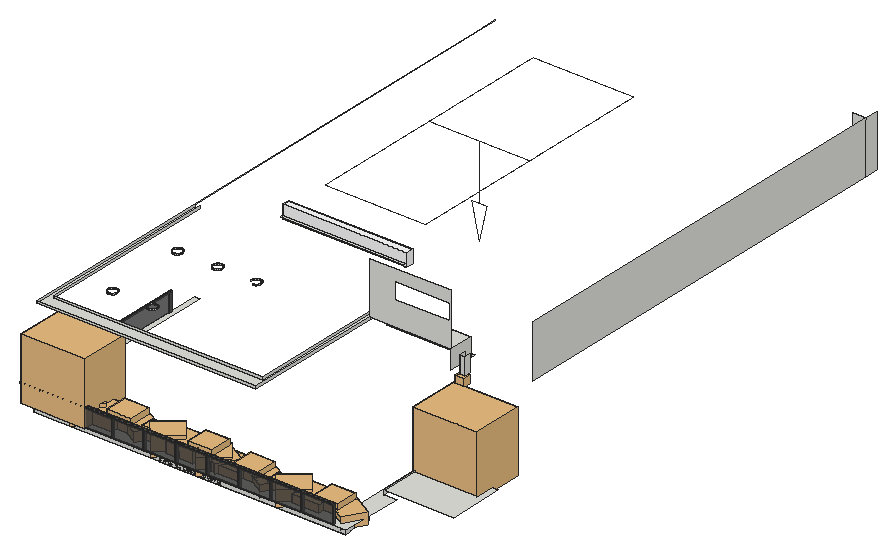
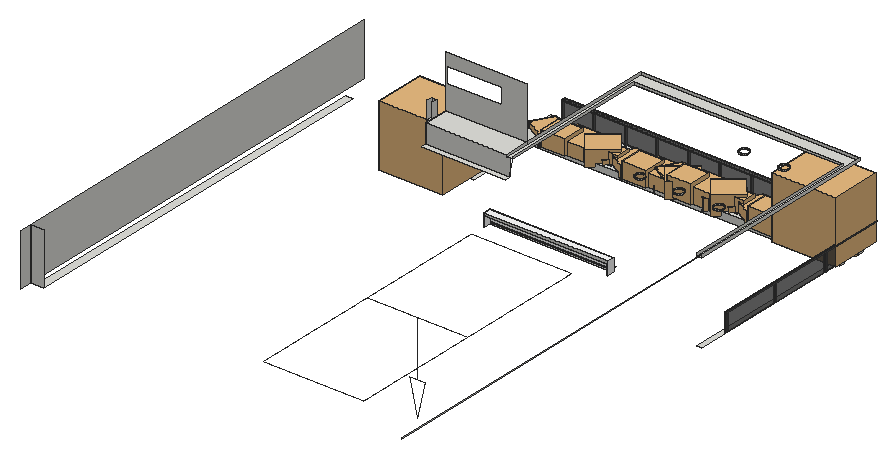
# SketchUp Ruby script. Lengths in inches.
U = 1.inch
M = Sketchup.active_model
def pt(a) = Geom::Point3d.new(a.map { |v| v * U })
def face(e, loops, mat)
  f = e.add_face(loops[0].map { |a| pt(a) })
  loops[1..].each { |l| e.add_face(l.map { |a| pt(a) }).erase! }
  f.material = f.back_material = mat if mat
  f
end
# faces: each face lists its corners as indices into pts; further lists are holes
def faces(e, pts, list, mat = nil) = list.each { |f| face(e, (f[0].is_a?(Array) ? f : [f]).map { |l| l.map { |i| pts[i] } }, mat) }
# xy, xz, yz: faces in a plane at the given z, y or x. An outline is a flat list of corners, or four numbers for a rectangle; further outlines are holes
def ring(l) = l.size == 4 ? [[l[0], l[1]], [l[2], l[1]], [l[2], l[3]], [l[0], l[3]]] : l.each_slice(2).to_a
def flat(e, list, mat, &to3) = list.each { |f| face(e, (f[0].is_a?(Array) ? f : [f]).map { |l| ring(l).map { |u, v| to3.(u, v) } }, mat) }
def xy(e, z, list, mat = nil) = flat(e, list, mat) { |x, y| [x, y, z] }
def xz(e, y, list, mat = nil) = flat(e, list, mat) { |x, z| [x, y, z] }
def yz(e, x, list, mat = nil) = flat(e, list, mat) { |y, z| [x, y, z] }
def lines(e, pts, list) = list.each { |a, b| e.add_line(pt(pts[a]), pt(pts[b])) }
# prism: a flat outline (further loops are holes) pulled along v
def prism(e, loops, v, mat = nil)
  f = face(e, loops, mat); d = Geom::Vector3d.new(v.map { |x| x * U })
  f.pushpull(f.normal.samedirection?(d) ? d.length : -d.length)
end
def box(e, o, s, mat = nil) = prism(e, [[o, [o[0] + s[0], o[1], o[2]], [o[0] + s[0], o[1] + s[1], o[2]], [o[0], o[1] + s[1], o[2]]]], [0, 0, s[2]], mat)
def at(x, y, z, deg = 0) = Geom::Transformation.translation(pt([x, y, z])) * Geom::Transformation.rotation(ORIGIN, Z_AXIS, deg.degrees)
def axes(o, x, y, z) = Geom::Transformation.new([*x, 0, *y, 0, *z, 0, *pt(o).to_a, 1])
def part(name) = M.definitions.add(name)
# library, detail: a bought-in or finely detailed component or shape, given as its bounding box
def library(name, o, s) = part(name).tap { |d| box(d.entities, o, s) }
def detail(e, o, s) = box(e.add_group.entities, o, s)
def put(e, d, t, mat = nil) = e.add_instance(d, t).tap { |i| i.material = mat if mat }
def group(e, t, mat = nil) = e.add_group.tap { |g| g.transformation = t; g.material = mat if mat }.entities
root = M.entities
M.materials.add("DefaultMaterial4").color = [255, 255, 255]
M.materials.add("Material__1").color = [95, 70, 46]
M.materials.add("[0135_DarkGray]").color = [81, 81, 81]
M.materials.add("[Translucent Glass Safety]").color = [204, 235, 244]
M.materials["[Translucent Glass Safety]"].alpha = 0.5
M.materials.add("[Translucent_Glass_Gray]1").color = [63, 63, 63]
M.materials["[Translucent_Glass_Gray]1"].alpha = 0.54
c1 = library("Areca palm plant",[0,0,0],[49.1,36.6,54.46])
c2 = library("Group38\#2",[14.01,28.44,-23.43],[18.58,18.32,38.89])
c3 = library("Group\#32",[-84.69,-90.07,-0.36],[176.51,175.13,171.4])
c4 = library("Group20\#1",[-20.81,-17.08,3.79],[39.86,39.43,37.51])
c5 = library("Group\#130",[-7.34,-1.2,0],[38.67,35.81,49.04])
c6 = part("Group\#35")
put(c6.entities,c1,axes([-6.2,158.41,6.08],[0.45017,-0.56191,0],[0.66137,0.52986,0],[0,0,0.72]))
put(c6.entities,c1,axes([-6.2,56.6,6.08],[0.45017,-0.56191,0],[0.66137,0.52986,0],[0,0,0.72]))
put(c6.entities,c2,axes([-4.1,-1.15,28.17],[0.8848,0,0],[0,0.94674,0],[0,0,0.85826]))
put(c6.entities,c2,axes([-4.1,100.66,28.17],[0.8848,0,0],[0,0.94674,0],[0,0,0.85826]))
g1 = group(c6.entities,at(0,0,0))
xy(g1,0,[[0,0,6,234.8],[30,0,36,234.8]])
xy(g1,3,[[6,0,30,234.8]])
xy(g1,7,[[6,5,30,229.8]],"Material__1")
xy(g1,15,[[[0,0,36,234.8],[6,5,30,229.8]]])
xz(g1,0,[[0,0,6,0,6,3,30,3,30,0,36,0,36,15,0,15]])
xz(g1,5,[[6,7,30,15]])
xz(g1,229.8,[[6,7,30,15]])
xz(g1,234.8,[[0,0,0,15,36,15,36,0,30,0,30,3,6,3,6,0]])
yz(g1,0,[[0,0,234.8,15]])
yz(g1,6,[[0,0,234.8,3],[5,7,229.8,15]])
yz(g1,30,[[0,0,234.8,3],[5,7,229.8,15]])
yz(g1,36,[[0,0,234.8,15]])
put(c6.entities,c3,axes([17.19,121.23,6.07],[-0.08133,-0.14087,0],[0.14087,-0.08133,0],[0,0,0.1725]))
put(c6.entities,c3,axes([14.93,173.12,6.05],[-0.04961,-0.08593,0],[0.08593,-0.04961,0],[0,0,0.10522]))
put(c6.entities,c4,axes([18.97,79.98,4.77],[0,0.85,0],[-0.85,0,0],[0,0,0.85]))
put(c6.entities,c3,axes([17.19,223.04,6.07],[-0.08133,-0.14087,0],[0.14087,-0.08133,0],[0,0,0.1725]))
put(c6.entities,c3,axes([14.93,71.3,6.05],[-0.04961,-0.08593,0],[0.08593,-0.04961,0],[0,0,0.10522]))
put(c6.entities,c5,axes([24.9375,191.72,8],[0,0.79,0],[-0.79,0,0],[0,0,0.79]))
put(c6.entities,c4,axes([18.97,181.79,4.77],[0,0.85,0],[-0.85,0,0],[0,0,0.85]))
put(c6.entities,c5,axes([24.9375,89.91,8],[0,0.79,0],[-0.79,0,0],[0,0,0.79]))
put(c6.entities,c3,axes([14.93,91.37,6.05],[-0.04961,-0.08593,0],[0.08593,-0.04961,0],[0,0,0.10522]))
put(c6.entities,c3,axes([14.93,145.87,6.05],[-0.04961,-0.08593,0],[0.08593,-0.04961,0],[0,0,0.10522]))
put(c6.entities,c3,axes([17.19,15.79,6.07],[-0.08133,-0.14087,0],[0.14087,-0.08133,0],[0,0,0.1725]))
put(c6.entities,c3,axes([14.93,193.18,6.05],[-0.04961,-0.08593,0],[0.08593,-0.04961,0],[0,0,0.10522]))
put(c6.entities,c3,axes([14.93,44.05,6.05],[-0.04961,-0.08593,0],[0.08593,-0.04961,0],[0,0,0.10522]))
c7 = part("Group72\#1")
p = [[0,0,0],[0,0,-70.14],[-9.72,0,-70.14],[63.31,-163.75,0],[-63.31,-163.75,0],[63.31,163.75,0],
  [63.31,0,0],[-63.31,163.75,0],[9.72,0,-70.14],[-63.31,0,0],[0,0,-113.53]]
lines(c7.entities,p,[[0,1],[1,2],[3,4],[5,6],[7,5],[1,8],[9,0],[0,6],[8,10],[4,9],[6,3],[2,10],
  [9,7]])
c8 = part("Rectangle Light")
put(c8.entities,c7,at(0,0,0))
c9 = library("Round Planter with Plant",[-35.48,-39.77,0],[80.62,63.55,77.875])
c10 = part("Group\#81")
box(c10.entities,[0,0,0],[0.79,39.37,35.43],"[Translucent_Glass_Gray]1")
c11 = part("Group\#82")
box(c11.entities,[0,0,0],[0.59,1.57,34.25])
c12 = part("Group\#85")
g2 = group(c12.entities,at(0.55,0.5,0))
put(g2,c10,axes([293.06,0,0],[0,0.84,0],[-0.92977,0,0],[0,0,1]),"[Translucent Glass Safety]")
g3 = group(g2,at(0,33.57,0),"[Translucent Glass Safety]")
box(g3,[0,0,0],[0.73,33.07,35.43],"[Translucent_Glass_Gray]1")
put(g2,c10,axes([218.38,0,0],[0,0.84,0],[-0.92977,0,0],[0,0,1]),"[Translucent Glass Safety]")
put(g2,c10,axes([367.73,0,0],[0,0.84,0],[-0.92977,0,0],[0,0,1]),"[Translucent Glass Safety]")
g4 = group(g2,at(31.69,0,0),"[Translucent Glass Safety]")
box(g4,[-30.96,0,0],[30.96,0.66,35.43],"[Translucent_Glass_Gray]1")
put(g2,c10,axes([255.72,0,0],[0,0.84,0],[-0.92977,0,0],[0,0,1]),"[Translucent Glass Safety]")
g5 = group(g2,at(181.04,0,0),"[Translucent Glass Safety]")
box(g5,[-36.61,0,0],[36.61,0.66,35.43],"[Translucent_Glass_Gray]1")
g6 = group(g2,at(0,0.66,0),"[Translucent Glass Safety]")
box(g6,[0,0,0],[0.73,32.24,35.43],"[Translucent_Glass_Gray]1")
g7 = group(g2,at(143.71,0,0),"[Translucent Glass Safety]")
box(g7,[-36.61,0,0],[36.61,0.66,35.43],"[Translucent_Glass_Gray]1")
g8 = group(g2,at(69.03,0,0),"[Translucent Glass Safety]")
box(g8,[-36.61,0,0],[36.61,0.66,35.43],"[Translucent_Glass_Gray]1")
g9 = group(g2,at(0,67.3,0),"[Translucent Glass Safety]")
box(g9,[0,0,0],[0.73,33.07,35.43],"[Translucent_Glass_Gray]1")
put(g2,c11,axes([107.44,0.66,0],[0,1,0],[-0.92977,0,0],[0,0,1]),"[0135_DarkGray]")
put(g2,c11,axes([144.78,0.66,0],[0,1,0],[-0.92977,0,0],[0,0,1]),"[0135_DarkGray]")
put(g2,c11,axes([182.11,0.66,0],[0,1,0],[-0.92977,0,0],[0,0,1]),"[0135_DarkGray]")
put(g2,c11,axes([256.79,0.66,0],[0,1,0],[-0.92977,0,0],[0,0,1]),"[0135_DarkGray]")
put(g2,c11,axes([368.14,0.66,0],[0,1,0],[-0.92977,0,0],[0,0,1]),"[0135_DarkGray]")
put(g2,c11,axes([0.73,98.83,0],[0.92977,0,0],[0,1,0],[0,0,1]),"[0135_DarkGray]")
put(g2,c11,axes([331.46,0.66,0],[0,1,0],[-0.92977,0,0],[0,0,1]),"[0135_DarkGray]")
g10 = group(g2,at(106.37,0,0),"[Translucent Glass Safety]")
box(g10,[-36.61,0,0],[36.61,0.66,35.43],"[Translucent_Glass_Gray]1")
put(g2,c10,axes([330.39,0,0],[0,0.84,0],[-0.92977,0,0],[0,0,1]),"[Translucent Glass Safety]")
put(g2,c11,axes([294.125,0.66,0],[0,1,0],[-0.92977,0,0],[0,0,1]),"[0135_DarkGray]")
put(g2,c11,axes([0.73,66.04,0],[0.92977,0,0],[0,1,0],[0,0,1]),"[0135_DarkGray]")
put(g2,c11,axes([0.73,32.31,0],[0.92977,0,0],[0,1,0],[0,0,1]),"[0135_DarkGray]")
put(g2,c11,axes([32.76,0.66,0],[0,1,0],[-0.92977,0,0],[0,0,1]),"[0135_DarkGray]")
put(g2,c11,axes([70.1,0.66,0],[0,1,0],[-0.92977,0,0],[0,0,1]),"[0135_DarkGray]")
put(g2,c11,axes([219.45,0.66,0],[0,1,0],[-0.92977,0,0],[0,0,1]),"[0135_DarkGray]")
g11 = group(c12.entities,at(0,0,34.25))
xy(g11,0,[[0,0,0,100.87,0.55,100.87,0.55,0.5,362.73,0.5,362.73,0],[362.73,0,369.35,0.5],[368.19,0.5,368.6875,1.16],[1.28,1.16,1.28,100.87,1.83,100.87,1.83,1.65,362.73,1.65,362.73,1.16],[362.73,1.16,368.19,1.65]],"[0135_DarkGray]")
xy(g11,1.18,[[368.19,0,368.6875,0.5],[368.6875,0,369.35,0.5],[0.55,0.5,0.55,100.87,1.28,100.87,1.28,1.16,362.73,1.16,362.73,0.5],[368.6875,0.5,369.35,1.16]],"[0135_DarkGray]")
xy(g11,1.97,[[0,0,362.73,0,362.73,1.65,1.83,1.65,1.83,100.87,0,100.87],[362.73,0,368.19,1.65]],"[0135_DarkGray]")
xz(g11,0,[[0,0,362.73,1.97],[362.73,0,369.35,0,369.35,1.18,368.19,1.18,368.19,1.97,362.73,1.97]],"[0135_DarkGray]")
xz(g11,0.5,[[0.55,0,1.28,1.18],[1.28,0,362.73,1.18],[362.73,0,368.19,1.18],[368.19,0,368.6875,1.18],[368.6875,0,369.35,1.18]],"[0135_DarkGray]")
xz(g11,1.16,[[1.28,0,362.73,1.18],[362.73,0,368.19,1.18]],"[0135_DarkGray]")
xz(g11,1.65,[[1.83,0,362.73,1.97],[362.73,0,368.19,1.97]],"[0135_DarkGray]")
xz(g11,100.87,[[0,0,0,1.97,1.83,1.97,1.83,0,1.28,0,1.28,1.18,0.55,1.18,0.55,0]],"[0135_DarkGray]")
yz(g11,0,[[0,0,100.87,1.97]],"[0135_DarkGray]")
yz(g11,0.55,[[0.5,0,100.87,1.18]],"[0135_DarkGray]")
yz(g11,1.28,[[1.16,0,100.87,1.18]],"[0135_DarkGray]")
yz(g11,1.83,[[1.65,0,100.87,1.97]],"[0135_DarkGray]")
yz(g11,362.73,[[0,0,0,1.97,1.65,1.97,1.65,0,1.16,0,1.16,1.18,0.5,1.18,0.5,0]],"[0135_DarkGray]")
yz(g11,368.19,[[1.16,0,1.65,0,1.65,1.97,0,1.97,0,1.18,1.16,1.18],[0.5,0,1.16,1.18]],"[0135_DarkGray]")
yz(g11,368.6875,[[0.5,0,1.16,1.18]],"[0135_DarkGray]")
yz(g11,369.35,[[0,0,0.5,1.18]],"[0135_DarkGray]")
c13 = library("Spot Light",[-5.1,-5.1,-11.05],[10.2,10.2,11.05])
c14 = part("Group\#68")
xy(c14.entities,48.43,[[59.06,0,59.06,5.91,59.65,5.91,59.65,0.59,138.39,0.59,138.39,5.91,138.98,5.91,138.98,0]],"DefaultMaterial4")
xy(c14.entities,53.9375,[[59.65,0.59,138.39,5.91]],"DefaultMaterial4")
xy(c14.entities,55.51,[[59.06,0,138.98,5.91]],"DefaultMaterial4")
xz(c14.entities,0,[[59.06,48.43,138.98,55.51]],"DefaultMaterial4")
xz(c14.entities,0.59,[[59.65,48.43,138.39,53.9375]],"DefaultMaterial4")
xz(c14.entities,5.91,[[59.06,48.43,59.06,55.51,138.98,55.51,138.98,48.43,138.39,48.43,138.39,53.9375,59.65,53.9375,59.65,48.43]])
yz(c14.entities,59.06,[[0,48.43,5.91,55.51]],"DefaultMaterial4")
yz(c14.entities,138.39,[[0.59,48.43,5.91,53.9375]],"DefaultMaterial4")
yz(c14.entities,138.98,[[0,48.43,5.91,55.51]],"DefaultMaterial4")
xy(root,273.1875,[[177.75,359.375,585.62,359.375,585.62,438.56,569.82,438.56,569.82,508.37,562.6875,508.37,562.6875,394.64,183.75,394.64,183.75,631.27,177.75,631.27]])
xy(root,278.125,[[569.82,438.56,657.75,508.37]])
xy(root,354.1875,[[449.19,593.57,554.88,600.32]])
xy(root,359.15,[[572.68,554.8125,578.99,562.125]])
xy(root,364.125,[[243.65,683.82,398.4,690.57]])
xy(root,375.25,[[177.75,383.3125,177.75,631.27,183.75,631.27,183.75,402.08,446,402.08,446,593.57,452.87,593.57,452.87,383.3125]])
xy(root,378,[[452.87,562.125,554.88,593.57],[641.5625,600.32,651,1087.125]])
xz(root,383.3125,[[177.75,375.25,452.87,378.5]])
xz(root,402.08,[[183.75,375.25,446,378]])
xz(root,554.8125,[[572.68,359.15,578.99,381.03]])
xz(root,562.125,[[[452.87,378,554.88,444],[484.27,408.9,554.02,429.22]]])
xz(root,593.57,[[449.43,354.1875,554.88,354.1875,554.88,378,452.87,378,452.87,375.25,449.43,375.25]])
xz(root,1087.125,[[641.5625,378,657.75,444]])
yz(root,177.75,[[383.3125,375.25,383.3125,378.5,1087.125,378.5,1087.125,378,631.27,378,631.27,375.25],[1087.125,378,1103.3125,378.5]])
yz(root,183.75,[[402.08,375.25,631.27,378]])
yz(root,446,[[402.08,375.25,593.57,378]])
yz(root,452.87,[[383.3125,375.25,562.125,378.5],[562.125,375.25,593.57,378]])
yz(root,554.88,[[562.125,354.1875,593.57,378]])
yz(root,569.82,[[438.56,273.1875,508.37,278.125]])
yz(root,572.68,[[554.8125,359.15,562.125,381.03]])
yz(root,578.99,[[554.8125,359.15,562.125,381.03]])
yz(root,657.75,[[562.125,378,1087.125,444],[1087.125,378,1103.3125,444]])
p = [[223.8125,438.06,378],[222.26,438.25,378],[222.26,438.25,379.1875],[223.8125,438.06,379.1875],[225.37,438.27,378],[225.37,438.27,379.1875],
  [274.1875,438.06,378],[272.63,438.25,378],[272.63,438.25,379.1875],[274.1875,438.06,379.1875],[275.74,438.27,378],[275.74,438.27,379.1875],
  [220.8125,438.85,378],[220.8125,438.85,379.1875],[226.81,438.87,378],[226.81,438.87,379.1875],[271.1875,438.85,378],[271.1875,438.85,379.1875],
  [277.19,438.87,378],[277.19,438.87,379.1875],[219.5625,439.8,378],[219.5625,439.8,379.1875],[269.9375,439.8,378],[269.9375,439.8,379.1875],
  [228.05,439.83,378],[228.05,439.83,379.1875],[278.42,439.83,378],[278.42,439.83,379.1875],[218.61,441.04,378],[218.61,441.04,379.1875],
  [229,441.08,378],[229,441.08,379.1875],[268.98,441.04,378],[268.98,441.04,379.1875],[279.375,441.08,378],[279.375,441.08,379.1875],
  [218,442.48,378],[218,442.48,379.1875],[268.375,442.48,378],[268.375,442.48,379.1875],[229.59,442.52,378],[229.59,442.52,379.1875],
  [279.97,442.52,378],[279.97,442.52,379.1875],[217.79,444.03,378],[217.79,444.03,379.1875],[229.79,444.08,378],[229.79,444.08,379.1875],
  [268.17,444.03,378],[268.17,444.03,379.1875],[280.17,444.08,378],[280.17,444.08,379.1875],[217.99,445.59,378],[217.99,445.59,379.1875],
  [268.36,445.59,378],[268.36,445.59,379.1875],[229.58,445.63,378],[229.58,445.63,379.1875],[279.96,445.63,378],[279.96,445.63,379.1875],
  [218.58,447.04,378],[218.58,447.04,379.1875],[228.98,447.08,378],[228.98,447.08,379.1875],[268.96,447.04,378],[268.96,447.04,379.1875],
  [279.35,447.08,378],[279.35,447.08,379.1875],[219.53,448.28,378],[219.53,448.28,379.1875],[269.91,448.28,378],[269.91,448.28,379.1875],
  [228.02,448.3125,378],[228.02,448.3125,379.1875],[278.39,448.3125,378],[278.39,448.3125,379.1875],[220.77,449.24,378],[220.77,449.24,379.1875],
  [226.77,449.26,378],[226.77,449.26,379.1875],[271.15,449.24,378],[271.15,449.24,379.1875],[277.15,449.26,378],[277.15,449.26,379.1875],
  [222.22,449.84,378],[222.22,449.84,379.1875],[272.59,449.84,378],[272.59,449.84,379.1875],[225.32,449.86,378],[225.32,449.86,379.1875],
  [275.7,449.86,378],[275.7,449.86,379.1875],[223.77,450.06,378],[223.77,450.06,379.1875],[274.14,450.06,378],[274.14,450.06,379.1875],
  [223.79,540.64,378],[222.24,540.85,378],[222.24,540.85,379.1875],[223.79,540.64,379.1875],[225.34,540.85,378],[225.34,540.85,379.1875],
  [274.17,540.64,378],[272.61,540.85,378],[272.61,540.85,379.1875],[274.17,540.64,379.1875],[275.72,540.85,378],[275.72,540.85,379.1875],
  [324.34,540.85,378],[322.79,540.64,378],[322.79,540.64,379.1875],[324.34,540.85,379.1875],[220.79,541.45,378],[220.79,541.45,379.1875],
  [226.79,541.45,378],[226.79,541.45,379.1875],[271.17,541.45,378],[271.17,541.45,379.1875],[277.17,541.45,378],[277.17,541.45,379.1875],
  [325.79,541.45,378],[325.79,541.45,379.1875],[219.55,542.4,378],[219.55,542.4,379.1875],[228.03,542.4,378],[228.03,542.4,379.1875],
  [269.92,542.4,378],[269.92,542.4,379.1875],[278.41,542.4,378],[278.41,542.4,379.1875],[327.03,542.4,378],[327.03,542.4,379.1875],
  [218.59,543.64,378],[218.59,543.64,379.1875],[228.99,543.64,378],[228.99,543.64,379.1875],[268.97,543.64,378],[268.97,543.64,379.1875],
  [279.36,543.64,378],[279.36,543.64,379.1875],[327.99,543.64,378],[327.99,543.64,379.1875],[217.99,545.09,378],[217.99,545.09,379.1875],
  [229.59,545.09,378],[229.59,545.09,379.1875],[268.37,545.09,378],[268.37,545.09,379.1875],[279.96,545.09,378],[279.96,545.09,379.1875],
  [328.59,545.09,378],[328.59,545.09,379.1875],[217.79,546.64,378],[217.79,546.64,379.1875],[229.79,546.64,378],[229.79,546.64,379.1875],
  [268.17,546.64,378],[268.17,546.64,379.1875],[280.17,546.64,378],[280.17,546.64,379.1875],[316.99,545.09,378],[316.79,546.64,378],
  [316.79,546.64,379.1875],[316.99,545.09,379.1875],[328.79,546.64,378],[328.79,546.64,379.1875],[217.99,548.2,378],[217.99,548.2,379.1875],
  [229.59,548.2,378],[229.59,548.2,379.1875],[268.37,548.2,378],[268.37,548.2,379.1875],[279.96,548.2,378],[279.96,548.2,379.1875],
  [316.99,548.2,378],[316.99,548.2,379.1875],[328.59,548.2,378],[328.59,548.2,379.1875],[218.59,549.64,378],[218.59,549.64,379.1875],
  [228.99,549.64,378],[228.99,549.64,379.1875],[268.97,549.64,378],[268.97,549.64,379.1875],[279.36,549.64,378],[279.36,549.64,379.1875],
  [317.59,549.64,378],[317.59,549.64,379.1875],[327.99,549.64,378],[327.99,549.64,379.1875],[219.55,550.89,378],[219.55,550.89,379.1875],
  [228.03,550.89,378],[228.03,550.89,379.1875],[269.92,550.89,378],[269.92,550.89,379.1875],[278.41,550.89,378],[278.41,550.89,379.1875],
  [318.55,550.89,378],[318.55,550.89,379.1875],[327.03,550.89,378],[327.03,550.89,379.1875],[220.79,551.84,378],[220.79,551.84,379.1875],
  [226.79,551.84,378],[226.79,551.84,379.1875],[271.17,551.84,378],[271.17,551.84,379.1875],[277.17,551.84,378],[277.17,551.84,379.1875],
  [319.79,551.84,378],[319.79,551.84,379.1875],[325.79,551.84,378],[325.79,551.84,379.1875],[222.24,552.4375,378],[222.24,552.4375,379.1875],
  [225.34,552.4375,378],[225.34,552.4375,379.1875],[272.61,552.4375,378],[272.61,552.4375,379.1875],[275.72,552.4375,378],[275.72,552.4375,379.1875],
  [321.24,552.4375,378],[321.24,552.4375,379.1875],[324.34,552.4375,378],[324.34,552.4375,379.1875],[223.79,552.64,378],[223.79,552.64,379.1875],
  [274.17,552.64,378],[274.17,552.64,379.1875],[322.79,552.64,378],[322.79,552.64,379.1875],[183.75,383.2,378],[183.75,383.3125,378],
  [452.87,593.57,378],[452.87,593.61,378],[449.92,594.8,354.69],[446,593.57,375.25]]
faces(root,p,[[0,1,2,3],[4,0,3,5],[6,7,8,9],[10,6,9,11],[1,12,13,2],[14,4,5,15],[7,16,17,8],[18,10,11,19],
  [12,20,21,13],[16,22,23,17],[24,14,15,25],[26,18,19,27],[20,28,29,21],[30,24,25,31],[22,32,33,23],[34,26,27,35],
  [28,36,37,29],[32,38,39,33],[40,30,31,41],[42,34,35,43],[36,44,45,37],[46,40,41,47],[38,48,49,39],[50,42,43,51],
  [44,52,53,45],[48,54,55,49],[56,46,47,57],[58,50,51,59],[52,60,61,53],[62,56,57,63],[54,64,65,55],[66,58,59,67],
  [60,68,69,61],[64,70,71,65],[72,62,63,73],[74,66,67,75],[68,76,77,69],[78,72,73,79],[70,80,81,71],[82,74,75,83],
  [76,84,85,77],[80,86,87,81],[88,78,79,89],[90,82,83,91],[84,92,93,85],[86,94,95,87],[92,88,89,93],[94,90,91,95],
  [96,97,98,99],[100,96,99,101],[102,103,104,105],[106,102,105,107],[108,109,110,111],[97,112,113,98],[114,100,101,115],[103,116,117,104],
  [118,106,107,119],[120,108,111,121],[112,122,123,113],[124,114,115,125],[116,126,127,117],[128,118,119,129],[130,120,121,131],[122,132,133,123],
  [134,124,125,135],[126,136,137,127],[138,128,129,139],[140,130,131,141],[132,142,143,133],[144,134,135,145],[136,146,147,137],[148,138,139,149],
  [150,140,141,151],[142,152,153,143],[154,144,145,155],[146,156,157,147],[158,148,149,159],[160,161,162,163],[164,150,151,165],[152,166,167,153],
  [168,154,155,169],[156,170,171,157],[172,158,159,173],[161,174,175,162],[176,164,165,177],[166,178,179,167],[180,168,169,181],[170,182,183,171],
  [184,172,173,185],[174,186,187,175],[188,176,177,189],[178,190,191,179],[192,180,181,193],[182,194,195,183],[196,184,185,197],[186,198,199,187],
  [200,188,189,201],[190,202,203,191],[204,192,193,205],[194,206,207,195],[208,196,197,209],[198,210,211,199],[212,200,201,213],[202,214,215,203],
  [216,204,205,217],[206,218,219,207],[220,208,209,221],[210,222,223,211],[224,212,213,225],[214,226,227,215],[226,216,217,227],[218,228,229,219],
  [228,220,221,229],[222,230,231,223],[230,224,225,231]])
lines(root,p,[[232,233],[234,235],[236,237]])
put(root,c6,axes([344.39,403.41,262.5],[0,-1,0],[1,0,0],[0,0,0.5]))
put(root,c6,axes([185.83,403.41,262.5],[0,-1,0],[1,0,0],[0,0,0.61]))
put(root,c8,axes([317.11,904.41,378.49],[-1,0,0],[0,1,0],[0,0,1]))
put(root,c9,at(603.78,526.35,272.9375))
put(root,c9,at(211.96,397.99,273.1875))
put(root,c12,axes([176.47,358.22,273.1875],[1.06496,0,0],[0,2.34,0],[0,0,0.67]))
put(root,c13,at(575.84,554.8125,359.14))
put(root,c14,axes([128.58,687.72,248.27],[1.94849,0,0],[0,1.4541,0],[0,0,2.31338]))
